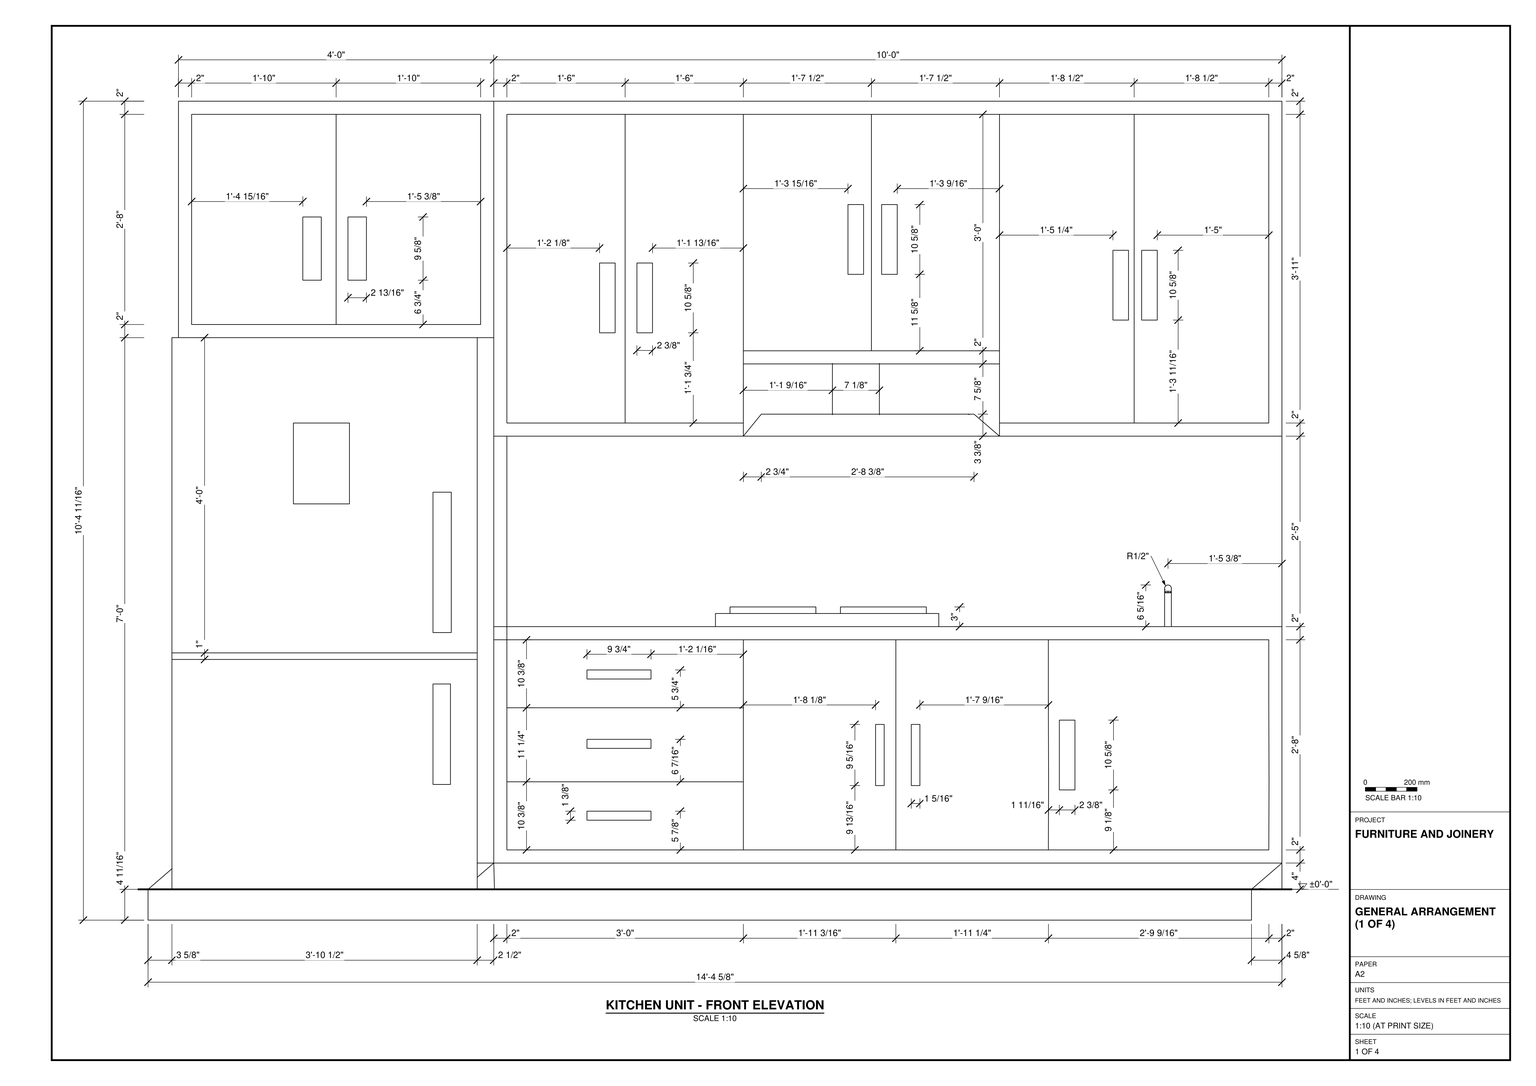
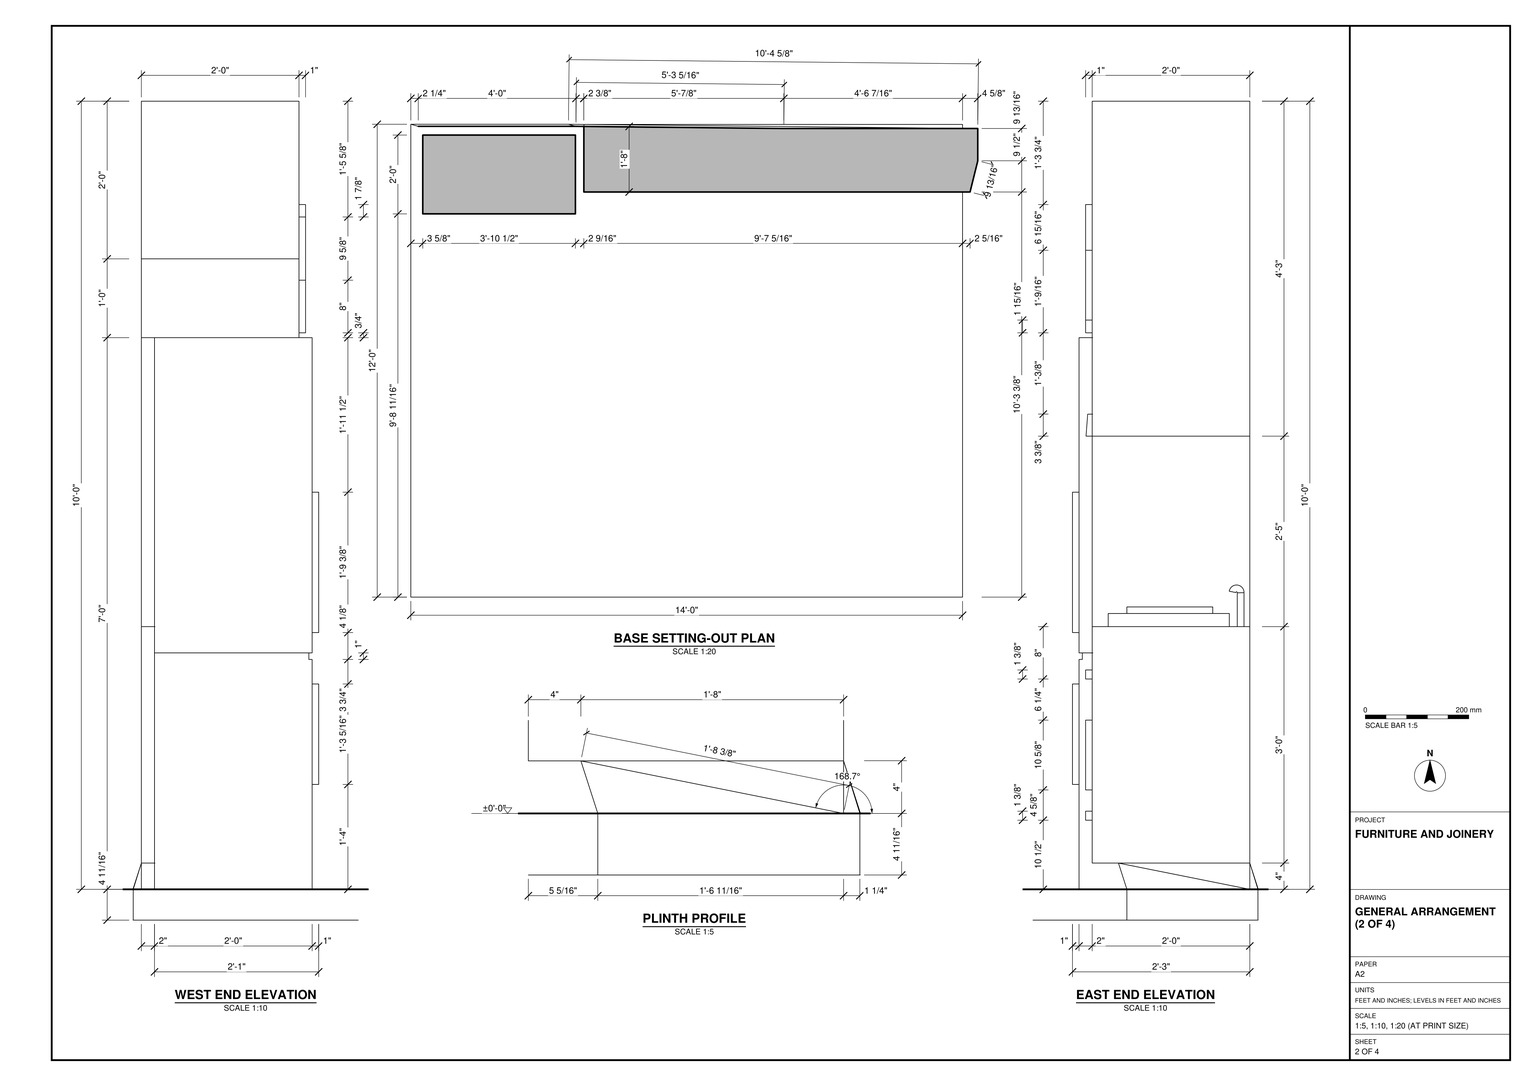
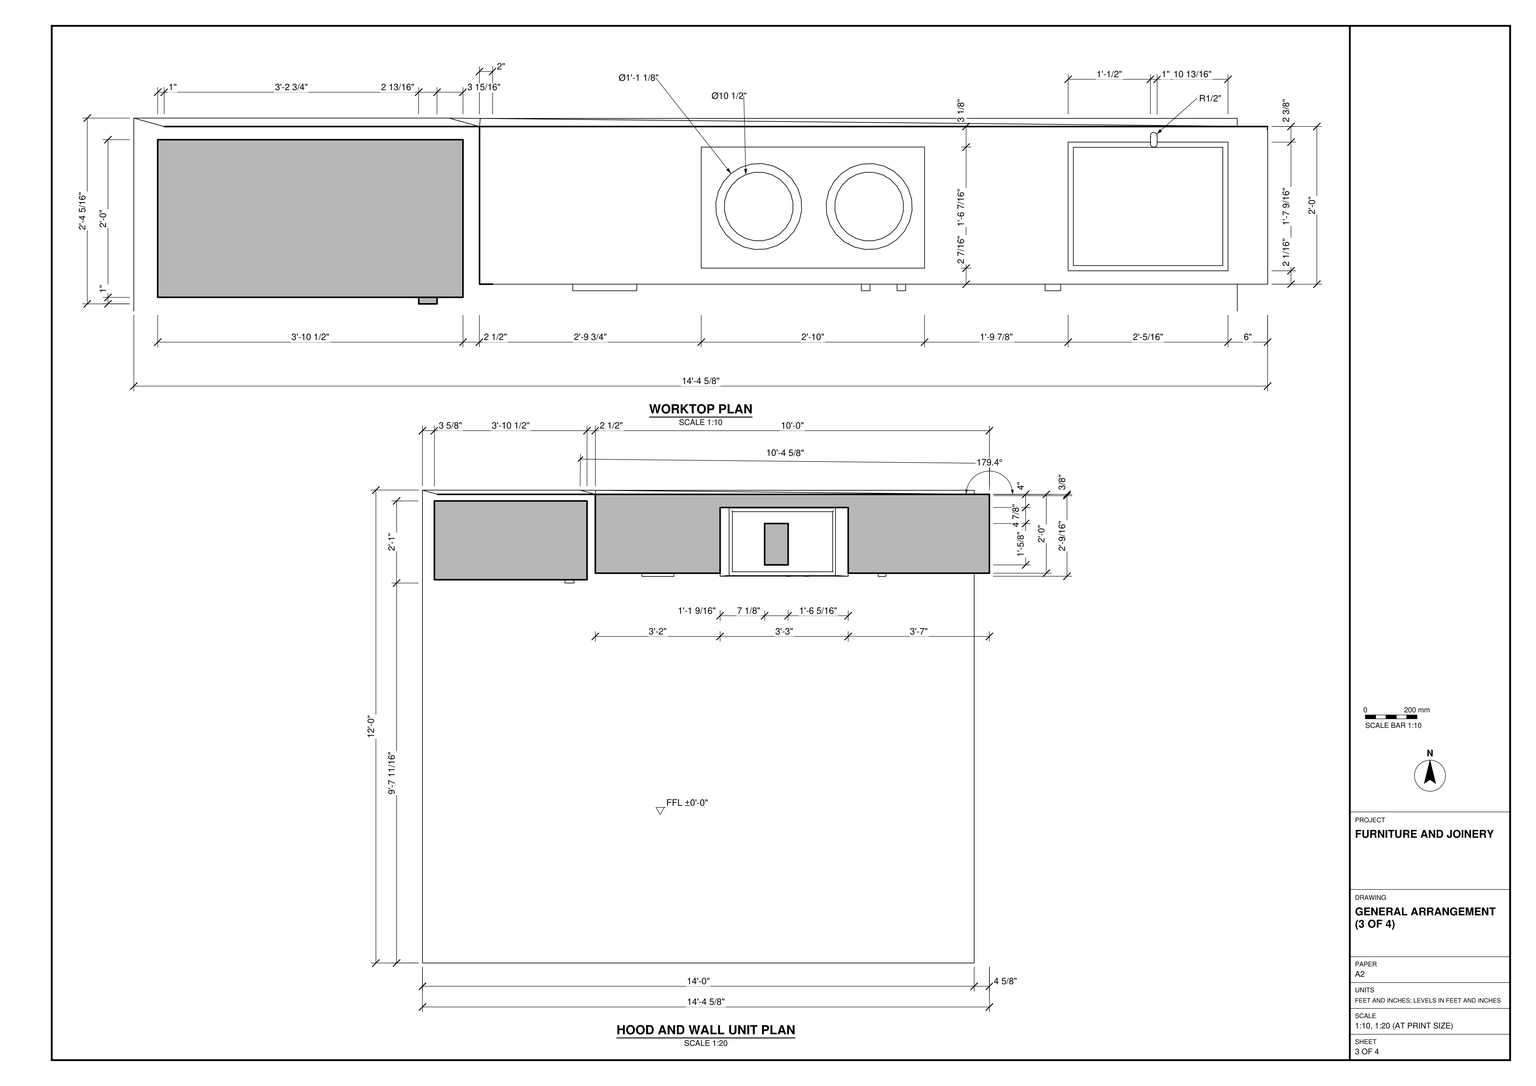
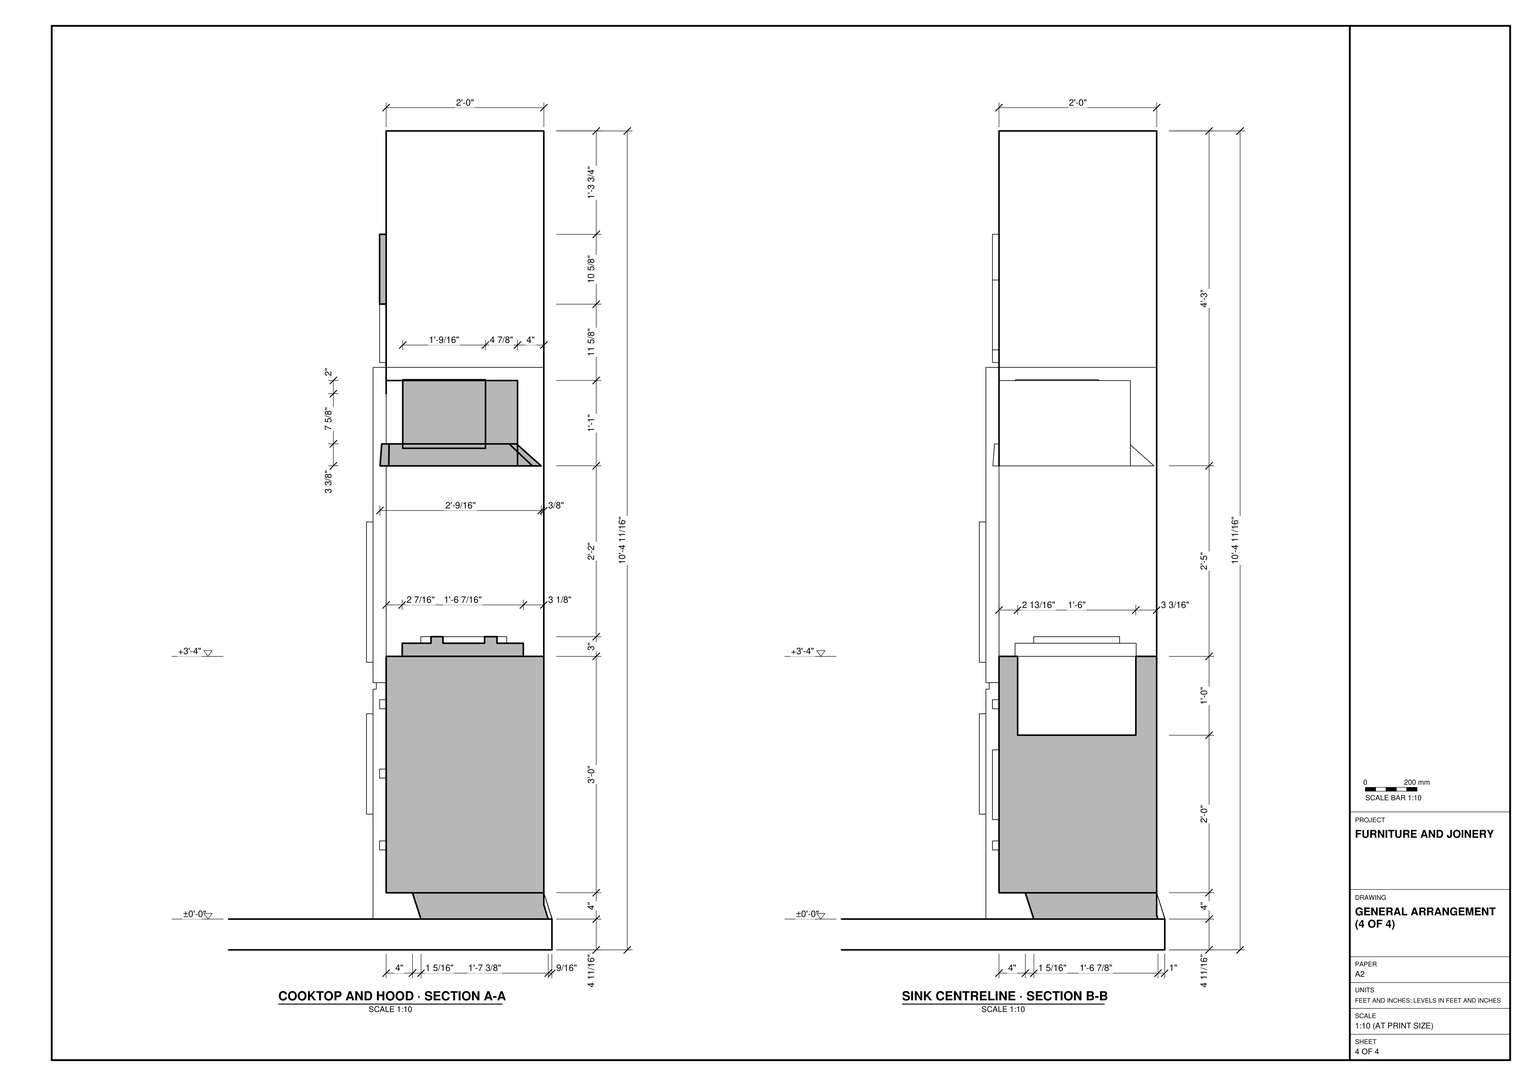
Build the kitchen unit in SketchUp from task_files/diagram_01.pdf. Work in feet and inches. The overall model is 14'-4 5/8" wide, 12'-0" deep and 10'-4 11/16" high, including the floor base. Use the single finished floor level of ±0'-0" as the datum. Set the cabinetry along the back edge of the floor base, leaving the floor in front clear.

Facing the unit, place the refrigerator on the left with a two-door cupboard above it. To its right, build the 10'-0" cabinet run on the plinth, following the sloping plinth profile in the end view. Below the worktop, place the drawer stack next to the refrigerator and the cupboard doors to the right. Follow the front elevation for the frame thicknesses, front divisions and pull positions. Fit the cooktop beneath the hood and the sink with its tap near the right end. Align the wall cupboard tops with the cupboard over the refrigerator, but shorten the middle pair of doors to leave space for the hood.

Keep the floor base and each joinery piece as separate groups or components, and use components for repeated parts such as matching pulls. Appliances, decor and loose items shown may be any suitable library components. Save one SketchUp model as output_files/kitchen_cabinet_run_with_its_worktop_and_appliances.skp.

# SketchUp Ruby script. Lengths in inches.
U = 1.inch
M = Sketchup.active_model
def pt(a) = Geom::Point3d.new(a.map { |v| v * U })
def face(e, loops, mat)
  f = e.add_face(loops[0].map { |a| pt(a) })
  loops[1..].each { |l| e.add_face(l.map { |a| pt(a) }).erase! }
  f.material = f.back_material = mat if mat
  f
end
# faces: each face lists its corners as indices into pts; further lists are holes
def faces(e, pts, list, mat = nil) = list.each { |f| face(e, (f[0].is_a?(Array) ? f : [f]).map { |l| l.map { |i| pts[i] } }, mat) }
# xy, xz, yz: faces in a plane at the given z, y or x. An outline is a flat list of corners, or four numbers for a rectangle; further outlines are holes
def ring(l) = l.size == 4 ? [[l[0], l[1]], [l[2], l[1]], [l[2], l[3]], [l[0], l[3]]] : l.each_slice(2).to_a
def flat(e, list, mat, &to3) = list.each { |f| face(e, (f[0].is_a?(Array) ? f : [f]).map { |l| ring(l).map { |u, v| to3.(u, v) } }, mat) }
def xy(e, z, list, mat = nil) = flat(e, list, mat) { |x, y| [x, y, z] }
def xz(e, y, list, mat = nil) = flat(e, list, mat) { |x, z| [x, y, z] }
def yz(e, x, list, mat = nil) = flat(e, list, mat) { |y, z| [x, y, z] }
def lines(e, pts, list) = list.each { |a, b| e.add_line(pt(pts[a]), pt(pts[b])) }
# prism: a flat outline (further loops are holes) pulled along v
def prism(e, loops, v, mat = nil)
  f = face(e, loops, mat); d = Geom::Vector3d.new(v.map { |x| x * U })
  f.pushpull(f.normal.samedirection?(d) ? d.length : -d.length)
end
def box(e, o, s, mat = nil) = prism(e, [[o, [o[0] + s[0], o[1], o[2]], [o[0] + s[0], o[1] + s[1], o[2]], [o[0], o[1] + s[1], o[2]]]], [0, 0, s[2]], mat)
def at(x, y, z, deg = 0) = Geom::Transformation.translation(pt([x, y, z])) * Geom::Transformation.rotation(ORIGIN, Z_AXIS, deg.degrees)
def axes(o, x, y, z) = Geom::Transformation.new([*x, 0, *y, 0, *z, 0, *pt(o).to_a, 1])
def part(name) = M.definitions.add(name)
# library, detail: a bought-in or finely detailed component or shape, given as its bounding box
def library(name, o, s) = part(name).tap { |d| box(d.entities, o, s) }
def detail(e, o, s) = box(e.add_group.entities, o, s)
def put(e, d, t, mat = nil) = e.add_instance(d, t).tap { |i| i.material = mat if mat }
def group(e, t, mat = nil) = e.add_group.tap { |g| g.transformation = t; g.material = mat if mat }.entities
root = M.entities
M.materials.add("[Color B08]").color = [102, 25, 0]
M.materials.add("[Color D01]").color = [255, 242, 204]
M.materials.add("[Color H08]").color = [0, 102, 102]
M.materials.add("[Color M06]").color = [86, 86, 86]
M.materials.add("[Color M08]").color = [30, 30, 30]
M.materials.add("[Color M09]").color = [0, 0, 0]
M.materials.add("[Marble Carrara Gold Floor Tile]").color = [225, 223, 217]
M.materials.add("[Wood Cherry Original]").color = [152, 86, 42]
xy(root,-4.6875,[[0,0,0,144,48,144,52.74,143.95,168,143.95,168,0]])
xy(root,0,[[0,0,168,0,168,124,52.74,124,52.74,143.95,48,144,0,144],[52.74,124,52.74,143.95,168,142.76,168,124],[168,124,168,142.76,172.64,142.71,169.26,129.1],[168,142.76,168,143.95,52.74,143.95]])
xy(root,4,[[52.64,118.71,172.64,122.71],[52.64,122.71,172.64,142.71]])
xy(root,10.53,[[66.83,117.71,76.58,118.71]],"[Color M09]")
xy(root,11.9,[[66.83,117.71,76.58,118.71]],"[Color M09]")
xy(root,15.14,[[138.75,117.71,141.125,118.71]],"[Color M09]")
xy(root,15.8,[[110.77,117.71,112.08,118.71],[116.21,117.71,117.52,118.71]],"[Color M09]")
xy(root,21.46,[[66.83,117.71,76.58,118.71]],"[Color M09]")
xy(root,22.84,[[66.83,117.71,76.58,118.71]],"[Color M09]")
xy(root,25.11,[[110.77,117.71,112.08,118.71],[116.21,117.71,117.52,118.71]],"[Color M09]")
xy(root,25.76,[[138.75,117.71,141.125,118.71]])
xy(root,28,[[143.05,121.55,165.8,139.55]])
xy(root,32.03,[[66.83,117.71,76.58,118.71]],"[Color M09]")
xy(root,33.4,[[66.83,117.71,76.58,118.71]],"[Color M09]")
xy(root,40,[[[142.25,120.75,166.59,140.34],[143.05,121.55,165.8,139.55]],[155.29,140.8,155.16,140.82,155.03,140.87,154.93,140.95,154.85,141.06,154.79,141.18,154.78,141.32,154.79,141.45,154.85,141.57,154.93,141.68,155.03,141.76,155.16,141.8125,155.29,141.83,155.42,141.8125,155.55,141.76,155.65,141.68,155.73,141.57,155.79,141.45,155.8,141.32,155.79,141.18,155.73,141.06,155.65,140.95,155.55,140.87,155.42,140.82]])
xy(root,40,[[[52.64,118.71,172.64,142.71],[142.25,120.75,166.59,140.34],[155.29,140.8,155.16,140.82,155.03,140.87,154.93,140.95,154.85,141.06,154.79,141.18,154.78,141.32,154.79,141.45,154.85,141.57,154.93,141.68,155.03,141.76,155.16,141.8125,155.29,141.83,155.42,141.8125,155.55,141.76,155.65,141.68,155.73,141.57,155.79,141.45,155.8,141.32,155.79,141.18,155.73,141.06,155.65,140.95,155.55,140.87,155.42,140.82]]],"[Marble Carrara Gold Floor Tile]")
xy(root,71.68,[[104.2,121.24,111.35,133.84]])
xy(root,82,[[90.64,118.71,129.64,138.71]])
xy(root,82.12,[[104.2,121.24,111.35,133.84]])
xy(root,84,[[4.64,118.71,52.64,142.71]])
xy(root,84.74,[[68.74,117.71,71.12,118.71],[74.43,117.71,76.81,118.71]],"[Color M09]")
xy(root,86.67,[[146.91,117.71,149.28,118.71],[151.28,117.71,153.66,118.71]],"[Color M09]")
xy(root,92.75,[[23.5625,117.71,26.375,118.71],[30.4375,117.71,33.25,118.71]],"[Color M09]")
xy(root,93.64,[[106.57,117.71,108.94,118.71],[111.69,117.71,114.07,118.71]],"[Color M09]")
xy(root,95.36,[[68.74,117.71,71.12,118.71],[74.43,117.71,76.81,118.71]],"[Color M09]")
xy(root,97.3,[[146.91,117.71,149.28,118.71],[151.28,117.71,153.66,118.71]],"[Color M09]")
xy(root,102.375,[[23.5625,117.71,26.375,118.71],[30.4375,117.71,33.25,118.71]],"[Color M09]")
xy(root,104.26,[[106.57,117.71,108.94,118.71],[111.69,117.71,114.07,118.71]],"[Color M09]")
xy(root,120,[[4.64,118.71,52.64,142.71],[52.64,118.71,172.64,142.71]],"[Color D01]")
xz(root,0,[[0,-4.6875,168,0]])
xz(root,117.71,[[66.83,10.53,76.58,11.9],[138.75,15.14,141.125,25.76],[110.77,15.8,112.08,25.11],[116.21,15.8,117.52,25.11],[66.83,21.46,76.58,22.84],
  [66.83,32.03,76.58,33.4],[68.74,84.74,71.12,95.36],[74.43,84.74,76.81,95.36],[146.91,86.67,149.28,97.3],[151.28,86.67,153.66,97.3],
  [23.5625,92.75,26.375,102.375],[30.4375,92.75,33.25,102.375],[106.57,93.64,108.94,104.26],[111.69,93.64,114.07,104.26]],"[Color M09]")
xz(root,118.71,[[66.83,10.53,76.58,11.9],[110.77,15.8,112.08,25.11],[116.21,15.8,117.52,25.11],[66.83,21.46,76.58,22.84],[66.83,32.03,76.58,33.4],
  [68.74,84.74,71.12,95.36],[74.43,84.74,76.81,95.36],[146.91,86.67,149.28,97.3],[106.57,93.64,108.94,104.26]])
xz(root,118.71,[[52.64,4,172.64,4,172.64,40,54.64,40,54.64,38,170.64,38,170.64,27.65,170.67,16.375,170.64,6,54.64,6,54.64,38,52.64,38],[52.64,69,90.64,69,90.64,71,54.64,71,54.64,118,170.64,118,170.64,71,129.64,71,129.64,69,172.64,69,172.64,120,52.64,120],[90.64,80,129.64,82],[[4.64,84,52.64,120],[6.64,86,50.64,118]]],"[Color B08]")
xz(root,118.71,[[[54.64,71,72.64,118],[68.74,84.74,71.12,95.36]],[[72.64,71,90.64,118],[74.43,84.74,76.81,95.36]],[[129.64,71,150.14,118],[146.91,86.67,149.28,97.3]],[[150.14,71,170.64,118],[151.28,86.67,153.66,97.3]],[[90.64,82,110.14,118],[106.57,93.64,108.94,104.26]],
  [[110.14,82,129.64,118],[111.69,93.64,114.07,104.26]],[[6.64,86,28.64,118],[23.5625,92.75,26.375,102.375]],[[28.64,86,50.64,118],[30.4375,92.75,33.25,102.375]]],"[Color D01]")
xz(root,118.71,[[[54.64,6,90.64,16.375],[66.83,10.53,76.58,11.9]],[[90.64,6,113.86,38],[110.77,15.8,112.08,25.11]],[[113.86,6,137.07,6,137.11,16.375,137.07,27.65,137.07,38,113.86,38],[116.21,15.8,117.52,25.11]],[[137.07,6,170.64,6,170.67,16.375,170.64,27.65,170.64,38,137.07,38,137.07,27.65,137.11,16.375],[138.75,15.14,141.125,25.76]],[[54.64,16.375,90.64,27.65],[66.83,21.46,76.58,22.84]],
  [[54.64,27.65,90.64,38],[66.83,32.03,76.58,33.4]]],"[Color H08]")
xz(root,118.71,[[52.64,38,54.64,40],[52.64,40,54.64,69]],"[Wood Cherry Original]")
xz(root,121.24,[[104.2,71.68,111.35,82.12]],"[Color M06]")
xz(root,121.55,[[143.05,28,165.8,40]])
xz(root,133.84,[[104.2,71.68,111.35,82.12]])
xz(root,138.71,[[90.64,69,129.64,82]],"[Color D01]")
xz(root,139.55,[[143.05,28,165.8,40]])
xz(root,142.71,[[172.64,0,52.64,4,172.64,4],[4.64,4,52.64,84],[52.64,4,172.64,40],[52.64,69,172.64,120],[4.64,84,52.64,120]])
xz(root,142.71,[[52.64,40,172.64,69]],"[Marble Carrara Gold Floor Tile]")
xz(root,143.95,[[52.74,-4.6875,168,0]])
xz(root,144,[[0,-4.6875,48,0]])
yz(root,0,[[0,-4.6875,144,0]])
yz(root,4.64,[[118.71,84,142.71,96],[118.71,96,142.71,120]],"[Color D01]")
yz(root,23.5625,[[117.71,92.75,118.71,102.375]],"[Color M09]")
yz(root,26.375,[[117.71,92.75,118.71,102.375]],"[Color M09]")
yz(root,30.4375,[[117.71,92.75,118.71,102.375]],"[Color M09]")
yz(root,33.25,[[117.71,92.75,118.71,102.375]],"[Color M09]")
yz(root,52.64,[[118.71,84,142.71,120]])
yz(root,52.64,[[118.71,4,142.71,40],[118.71,40,142.71,84]],"[Wood Cherry Original]")
yz(root,66.83,[[117.71,10.53,118.71,11.9],[117.71,21.46,118.71,22.84],[117.71,32.03,118.71,33.4]],"[Color M09]")
yz(root,68.74,[[117.71,84.74,118.71,95.36]],"[Color M09]")
yz(root,71.12,[[117.71,84.74,118.71,95.36]],"[Color M09]")
yz(root,74.43,[[117.71,84.74,118.71,95.36]])
yz(root,76.58,[[117.71,10.53,118.71,11.9],[117.71,21.46,118.71,22.84],[117.71,32.03,118.71,33.4]],"[Color M09]")
yz(root,76.81,[[117.71,84.74,118.71,95.36]],"[Color M09]")
yz(root,90.64,[[118.71,69,138.71,82]],"[Color D01]")
yz(root,104.2,[[121.24,71.68,133.84,82.12]])
yz(root,106.57,[[117.71,93.64,118.71,104.26]],"[Color M09]")
yz(root,108.94,[[117.71,93.64,118.71,104.26]],"[Color M09]")
yz(root,110.77,[[117.71,15.8,118.71,25.11]],"[Color M09]")
yz(root,111.35,[[121.24,71.68,133.84,82.12]])
yz(root,111.69,[[117.71,93.64,118.71,104.26]],"[Color M09]")
yz(root,112.08,[[117.71,15.8,118.71,25.11]],"[Color M09]")
yz(root,114.07,[[117.71,93.64,118.71,104.26]],"[Color M09]")
yz(root,116.21,[[117.71,15.8,118.71,25.11]],"[Color M09]")
yz(root,117.52,[[117.71,15.8,118.71,25.11]],"[Color M09]")
yz(root,129.64,[[118.71,69,138.71,82]],"[Color D01]")
yz(root,138.75,[[117.71,15.14,118.71,25.76]],"[Color M09]")
yz(root,141.125,[[117.71,15.14,118.71,25.76]],"[Color M09]")
yz(root,143.05,[[121.55,28,139.55,40]])
yz(root,146.91,[[117.71,86.67,118.71,97.3]],"[Color M09]")
yz(root,149.28,[[117.71,86.67,118.71,97.3]],"[Color M09]")
yz(root,151.28,[[117.71,86.67,118.71,97.3]],"[Color M09]")
yz(root,153.66,[[117.71,86.67,118.71,97.3]],"[Color M09]")
yz(root,165.8,[[121.55,28,139.55,40]])
yz(root,168,[[0,-4.6875,124,0],[124,-4.6875,143.95,0]])
yz(root,172.64,[[118.71,69,142.71,120]])
yz(root,172.64,[[142.71,0,142.71,4,122.71,4],[118.71,4,142.71,40]],"[Wood Cherry Original]")
p = [[48,144,0],[52.74,143.95,0],[52.74,143.95,-4.6875],[48,144,-4.6875],[172.64,122.71,4],[52.64,122.71,4],
  [52.74,124,0],[168,124,0],[52.64,142.71,4],[169.26,129.1,0],[172.64,142.71,0],[0,144,0],
  [4.64,142.71,4],[168,142.76,0],[155.03,140.87,40],[155.16,140.82,40],[155.16,140.82,45.15],[155.03,140.87,45.15],
  [155.29,140.8,40],[155.29,140.8,45.15],[155.42,140.82,40],[155.42,140.82,45.15],[155.55,140.87,40],[155.55,140.87,45.15],
  [154.93,140.95,40],[154.93,140.95,45.15],[155.65,140.95,40],[155.65,140.95,45.15],[154.85,141.06,40],[154.85,141.06,45.16],
  [155.73,141.06,40],[155.73,141.06,45.16],[154.79,141.18,40],[154.79,141.18,45.16],[155.79,141.18,40],[155.79,141.18,45.16],
  [154.78,141.32,40],[154.78,141.32,45.16],[155.8,141.32,40],[155.8,141.32,45.16],[154.79,141.45,40],[154.79,141.45,45.17],
  [155.79,141.45,40],[155.79,141.45,45.17],[154.85,141.57,40],[154.85,141.57,45.17],[155.73,141.57,40],[155.73,141.57,45.17],
  [154.93,141.68,40],[154.93,141.68,45.17],[155.65,141.68,40],[155.65,141.68,45.17],[155.03,141.76,40],[155.03,141.76,45.18],
  [155.55,141.76,40],[155.55,141.76,45.18],[155.16,141.8125,40],[155.16,141.8125,45.18],[155.29,141.83,40],[155.29,141.83,45.18],
  [155.42,141.8125,40],[155.42,141.8125,45.18],[155.16,140.8125,45.23],[155.03,140.87,45.24],[155.29,140.8,45.23],[155.42,140.8125,45.23],
  [155.55,140.87,45.24],[154.93,140.95,45.26],[155.65,140.95,45.26],[154.93,140.4375,45.22],[155.03,140.52,45.2],[155.16,140.57,45.19],
  [155.29,140.59,45.1875],[155.42,140.57,45.19],[155.55,140.52,45.2],[155.65,140.4375,45.22],[155.73,140.33,45.24],[155.79,140.21,45.26],
  [155.8,140.08,45.29],[155.79,139.95,45.32],[155.73,139.83,45.34],[155.65,139.73,45.36],[155.55,139.65,45.38],[155.42,139.6,45.39],
  [155.29,139.58,45.39],[155.16,139.6,45.39],[155.03,139.65,45.38],[154.93,139.73,45.36],[154.85,139.83,45.34],[154.79,139.95,45.32],
  [154.78,140.08,45.29],[154.79,140.21,45.26],[154.85,140.33,45.24],[154.79,140.23,45.37],[154.85,140.35,45.32],[155.73,140.35,45.32],
  [155.79,140.23,45.37],[154.93,140.45,45.29],[155.65,140.45,45.29],[155.03,140.53,45.26],[155.55,140.53,45.26],[155.03,140.55,45.3],
  [155.16,140.59,45.27],[155.16,140.58,45.25],[155.42,140.59,45.27],[155.55,140.55,45.3],[155.42,140.58,45.25],[155.29,140.61,45.26],
  [155.29,140.6,45.24],[155.16,140.8,45.26],[155.03,140.85,45.28],[155.29,140.79,45.25],[155.42,140.8,45.26],[155.55,140.85,45.28],
  [154.85,141.05,45.28],[154.93,140.92,45.32],[155.65,140.92,45.32],[155.73,141.05,45.28],[154.79,141.17,45.3],[155.79,141.17,45.3],
  [154.78,141.31,45.33],[155.8,141.31,45.33],[154.79,141.4375,45.35],[155.79,141.4375,45.35],[154.85,141.56,45.375],[155.73,141.56,45.375],
  [154.93,141.66,45.4],[155.65,141.66,45.4],[155.03,141.75,45.41],[155.16,141.8,45.42],[155.42,141.8,45.42],[155.55,141.75,45.41],
  [155.29,141.8125,45.42],[154.93,139.76,45.53],[154.85,139.86,45.49],[155.73,139.86,45.49],[155.65,139.76,45.53],[154.79,139.98,45.45],
  [155.79,139.98,45.45],[154.78,140.11,45.41],[155.8,140.11,45.41],[154.79,140.29,45.48],[154.85,140.39,45.41],[155.73,140.39,45.41],
  [155.79,140.29,45.48],[154.85,140.46,45.48],[154.93,140.53,45.4],[154.93,140.48,45.35],[155.65,140.53,45.4],[155.73,140.46,45.48],
  [155.65,140.48,45.35],[154.93,140.58,45.4375],[155.03,140.62,45.36],[155.03,140.58,45.34],[155.55,140.62,45.36],[155.65,140.58,45.4375],
  [155.55,140.58,45.34],[155.03,140.66,45.375],[155.16,140.67,45.33],[155.16,140.64,45.32],[155.16,140.62,45.3],[155.29,140.67,45.31],
  [155.29,140.65,45.3],[155.29,140.625,45.29],[155.42,140.67,45.33],[155.42,140.64,45.32],[155.42,140.62,45.3],[155.55,140.66,45.375],
  [155.03,140.79,45.35],[155.16,140.76,45.31],[155.16,140.73,45.32],[155.03,140.75,45.37],[155.16,140.7,45.33],[155.03,140.71,45.38],
  [155.29,140.75,45.29],[155.29,140.73,45.31],[155.29,140.7,45.3125],[155.42,140.76,45.31],[155.42,140.73,45.32],[155.42,140.7,45.33],
  [155.55,140.79,45.35],[155.55,140.75,45.37],[155.55,140.71,45.38],[155.03,140.83,45.32],[154.93,140.89,45.375],[154.93,140.84,45.42],
  [155.16,140.79,45.29],[155.29,140.77,45.28],[155.42,140.79,45.29],[155.55,140.83,45.32],[155.65,140.89,45.375],[155.65,140.84,45.42],
  [154.85,141.02,45.37],[154.85,140.97,45.44],[155.73,141.02,45.37],[155.73,140.97,45.44],[154.79,141.13,45.42],[155.79,141.13,45.42],
  [154.78,141.25,45.48],[155.8,141.25,45.48],[154.79,141.375,45.54],[155.79,141.375,45.54],[155.03,139.68,45.55],[155.16,139.63,45.57],
  [155.29,139.62,45.58],[155.42,139.63,45.57],[155.55,139.68,45.55],[154.79,140.07,45.63],[154.78,140.18,45.55],[155.8,140.18,45.55],
  [155.79,140.07,45.63],[154.79,140.375,45.57],[155.79,140.375,45.57],[154.85,140.625,45.5625],[154.93,140.65,45.46],[154.85,140.54,45.53],
  [155.65,140.65,45.46],[155.73,140.625,45.5625],[155.73,140.54,45.53],[154.93,140.71,45.46],[155.65,140.71,45.46],[154.85,140.8125,45.55],
  [154.93,140.78,45.45],[154.85,140.72,45.57],[155.65,140.78,45.45],[155.73,140.8125,45.55],[155.73,140.72,45.57],[154.85,140.9,45.51],
  [155.73,140.9,45.51],[154.79,141.0625,45.53],[154.79,140.97,45.61],[155.79,141.0625,45.53],[155.79,140.97,45.61],[154.78,141.16,45.61],
  [155.8,141.16,45.61],[154.85,141.49,45.59],[155.73,141.49,45.59],[154.93,141.58,45.64],[155.65,141.58,45.64],[155.03,141.66,45.68],
  [155.55,141.66,45.68],[155.16,141.7,45.7],[155.29,141.72,45.71],[155.42,141.7,45.7],[155.03,139.81,45.81],[154.93,139.875,45.76],
  [155.65,139.875,45.76],[155.55,139.81,45.81],[154.85,139.96,45.7],[155.73,139.96,45.7],[154.78,140.29,45.68],[155.8,140.29,45.68],
  [154.79,140.48,45.65],[155.79,140.48,45.65],[154.79,140.6,45.6875],[155.79,140.6,45.6875],[154.79,140.85,45.67],[154.79,140.73,45.69],
  [155.79,140.85,45.67],[155.79,140.73,45.69],[154.78,141.04,45.72],[155.8,141.04,45.72],[154.79,141.27,45.7],[155.79,141.27,45.7],
  [154.85,141.36,45.78],[155.73,141.36,45.78],[155.16,139.76,45.83],[155.29,139.75,45.84],[155.42,139.76,45.83],[154.85,140.12,45.87],
  [154.79,140.2,45.78],[155.79,140.2,45.78],[155.73,140.12,45.87],[154.78,140.42,45.77],[155.8,140.42,45.77],[154.78,140.58,45.82],
  [155.8,140.58,45.82],[154.78,140.9,45.79],[155.8,140.9,45.79],[154.79,141.12,45.83],[155.79,141.12,45.83],[154.93,141.44,45.86],
  [155.03,141.5,45.91],[155.55,141.5,45.91],[155.65,141.44,45.86],[154.93,140.05,45.95],[155.65,140.05,45.95],[154.79,140.36,45.89],
  [155.79,140.36,45.89],[154.78,140.74,45.83],[155.8,140.74,45.83],[154.79,140.94,45.92],[155.79,140.94,45.92],[154.85,141.1875,45.9375],
  [155.73,141.1875,45.9375],[155.16,141.54,45.94],[155.29,141.55,45.95],[155.42,141.54,45.94],[155.29,139.95,46.07],[155.16,139.96,46.05],
  [155.42,139.96,46.05],[155.03,139.99,46.01],[155.55,139.99,46.01],[154.85,140.31,46],[155.73,140.31,46],[154.79,140.55,45.95],
  [155.79,140.55,45.95],[154.79,140.75,45.96],[155.79,140.75,45.96],[154.85,140.98,46.04],[155.73,140.98,46.04],[154.93,141.25,46.03],
  [155.65,141.25,46.03],[154.93,140.26,46.09],[155.65,140.26,46.09],[154.85,140.53,46.07],[155.73,140.53,46.07],[154.85,140.76,46.09],
  [155.73,140.76,46.09],[154.93,141.02,46.14],[155.65,141.02,46.14],[155.03,141.29,46.09],[155.55,141.29,46.09],[155.16,141.32,46.14],
  [155.29,141.33,46.15],[155.42,141.32,46.14],[155.03,140.23,46.17],[155.16,140.2,46.22],[155.55,140.23,46.17],[155.42,140.2,46.22],
  [154.93,140.51,46.18],[155.65,140.51,46.18],[154.93,140.76,46.19],[155.65,140.76,46.19],[155.03,141.04,46.22],[155.55,141.04,46.22],
  [155.29,140.19,46.23],[155.03,140.49,46.26],[155.55,140.49,46.26],[155.03,140.77,46.27],[155.55,140.77,46.27],[155.16,141.06,46.27],
  [155.42,141.06,46.27],[155.29,141.07,46.28],[155.16,140.48,46.31],[155.29,140.48,46.33],[155.42,140.48,46.31],[155.16,140.77,46.33],
  [155.42,140.77,46.33],[155.29,140.77,46.34],[4.64,142.71,0],[155.29,141.32,40],[155.29,141.32,45.16],[155.29,141.31,45.33],
  [155.29,141.25,45.48],[155.29,141.16,45.61],[155.29,141.04,45.72],[155.29,140.9,45.79],[155.29,140.74,45.83],[155.29,140.58,45.82],
  [155.29,140.42,45.77],[155.29,140.29,45.68],[155.29,140.18,45.55],[155.29,140.11,45.41],[155.29,140.07,45.25],[155.29,141.32,45.25]]
faces(root,p,[[0,1,2,3],[8,1,6,5],[9,10,4,7],[11,12,8,0],[0,8,1],[13,1,8,10],[14,15,16,17],[15,18,19,16],
  [18,20,21,19],[20,22,23,21],[24,14,17,25],[22,26,27,23],[28,24,25,29],[26,30,31,27],[32,28,29,33],[30,34,35,31],
  [36,32,33,37],[34,38,39,35],[40,36,37,41],[38,42,43,39],[44,40,41,45],[42,46,47,43],[48,44,45,49],[46,50,51,47],
  [52,48,49,53],[50,54,55,51],[56,52,53,57],[58,56,57,59],[60,58,59,61],[54,60,61,55],[17,16,62,63],[16,19,64,62],
  [19,21,65,64],[21,23,66,65],[25,17,63,67],[23,27,68,66],[69,70,71,72,73,74,75,76,77,78,79,80,81,82,83,84,85,86,87,88,89,90,91,92],[93,94,92,91],[95,96,77,76],[94,97,69,92],
  [98,95,76,75],[97,99,70,69],[100,98,75,74],[101,102,103,99],[99,103,71,70],[104,105,100,106],[106,100,74,73],[102,107,108,103],
  [103,108,72,71],[107,104,106,108],[108,106,73,72],[63,62,109,110],[62,64,111,109],[64,65,112,111],[65,66,113,112],[29,25,67,114],
  [67,63,110,115],[66,68,116,113],[27,31,117,68],[33,29,114,118],[31,35,119,117],[37,33,118,120],[35,39,121,119],[41,37,120,122],
  [39,43,123,121],[45,41,122,124],[43,47,125,123],[49,45,124,126],[47,51,127,125],[53,49,126,128],[57,53,128,129],[55,61,130,131],
  [51,55,131,127],[59,57,129,132],[61,59,132,130],[133,134,88,87],[135,136,81,80],[134,137,89,88],[138,135,80,79],[137,139,90,89],
  [140,138,79,78],[139,93,91,90],[96,140,78,77],[141,142,94,93],[143,144,96,95],[145,146,147,142],[142,147,97,94],[148,149,143,150],
  [150,143,95,98],[151,152,153,146],[146,153,101,147],[147,101,99,97],[154,155,148,156],[156,148,150,105],[105,150,98,100],[157,158,159,152],
  [152,159,160,153],[153,160,102,101],[158,161,162,159],[159,162,163,160],[160,163,107,102],[161,164,165,162],[162,165,166,163],[163,166,104,107],
  [164,167,154,165],[165,154,156,166],[166,156,105,104],[168,169,170,171],[171,170,172,173],[173,172,158,157],[169,174,175,170],[170,175,176,172],
  [172,176,161,158],[174,177,178,175],[175,178,179,176],[176,179,164,161],[177,180,181,178],[178,181,182,179],[179,182,167,164],[115,110,183,184],
  [184,183,168,185],[110,109,186,183],[183,186,169,168],[109,111,187,186],[186,187,174,169],[111,112,188,187],[187,188,177,174],[112,113,189,188],
  [188,189,180,177],[113,116,190,189],[189,190,191,180],[114,67,115,192],[192,115,184,193],[68,117,194,116],[116,194,195,190],[118,114,192,196],
  [117,119,197,194],[120,118,196,198],[119,121,199,197],[122,120,198,200],[121,123,201,199],[202,133,87,86],[203,202,86,85],[204,203,85,84],
  [205,204,84,83],[206,205,83,82],[136,206,82,81],[207,208,139,137],[209,210,138,140],[208,141,93,139],[144,209,140,96],[211,145,142,141],
  [149,212,144,143],[213,214,151,215],[215,151,146,145],[216,217,218,155],[155,218,149,148],[219,173,157,214],[214,157,152,151],[182,220,216,167],
  [167,216,155,154],[221,222,219,223],[222,171,173,219],[181,224,220,182],[224,225,226,220],[193,184,185,227],[227,185,222,221],[185,168,171,222],
  [180,191,224,181],[190,195,228,191],[191,228,225,224],[229,193,227,230],[195,231,232,228],[196,192,193,229],[194,197,231,195],[198,196,229,233],
  [197,199,234,231],[124,122,200,235],[123,125,236,201],[126,124,235,237],[125,127,238,236],[128,126,237,239],[127,131,240,238],[129,128,239,241],
  [132,129,241,242],[130,132,242,243],[131,130,243,240],[244,245,133,202],[246,247,206,136],[245,248,134,133],[249,246,136,135],[248,207,137,134],
  [210,249,135,138],[250,211,141,208],[212,251,209,144],[252,215,145,211],[218,253,212,149],[254,213,215,252],[217,255,253,218],[223,219,214,213],
  [220,226,217,216],[256,221,223,257],[225,258,259,226],[230,227,221,256],[228,232,258,225],[233,229,230,260],[231,234,261,232],[200,198,233,262],
  [199,201,263,234],[235,200,262,264],[201,236,265,263],[266,244,202,203],[267,266,203,204],[268,267,204,205],[247,268,205,206],[269,270,207,248],
  [271,272,249,210],[270,250,208,207],[251,271,210,209],[273,252,211,250],[253,274,251,212],[275,254,252,273],[255,276,274,253],[257,223,213,254],
  [226,259,255,217],[260,230,256,277],[232,261,278,258],[262,233,260,279],[234,263,280,261],[237,235,264,281],[239,237,281,282],[238,240,283,284],
  [236,238,284,265],[285,269,248,245],[272,286,246,249],[287,273,250,270],[274,288,271,251],[289,257,254,275],[259,290,276,255],[277,256,257,289],
  [258,278,290,259],[279,260,277,291],[261,280,292,278],[264,262,279,293],[263,265,294,280],[241,239,282,295],[242,241,295,296],[243,242,296,297],
  [240,243,297,283],[298,299,266,267],[300,298,267,268],[301,285,245,244],[299,301,244,266],[302,300,268,247],[286,302,247,246],[303,287,270,269],
  [288,304,272,271],[305,275,273,287],[276,306,288,274],[307,289,275,305],[290,308,306,276],[291,277,289,307],[278,292,308,290],[293,279,291,309],
  [280,294,310,292],[281,264,293,311],[265,284,312,294],[313,303,269,285],[304,314,286,272],[315,305,287,303],[306,316,304,288],[317,307,305,315],
  [308,318,316,306],[309,291,307,317],[292,310,318,308],[311,293,309,319],[294,312,320,310],[282,281,311,321],[284,283,322,312],[295,282,321,323],
  [296,295,323,324],[297,296,324,325],[283,297,325,322],[326,313,285,301],[327,326,301,299],[328,329,300,302],[314,328,302,286],[330,315,303,313],
  [316,331,314,304],[319,309,317,332],[310,320,333,318],[321,311,319,334],[312,322,335,320],[336,327,299,298],[329,336,298,300],[337,330,313,326],
  [331,338,328,314],[332,317,315,330],[318,333,331,316],[334,319,332,339],[320,335,340,333],[323,321,334,341],[322,325,342,335],[324,323,341,343],
  [325,324,343,342],[344,337,326,327],[345,344,327,336],[346,345,336,329],[338,346,329,328],[339,332,330,337],[333,340,338,331],[341,334,339,347],
  [335,342,348,340],[347,339,337,344],[349,347,344,345],[348,349,345,346],[340,348,346,338],[343,341,347,349],[342,343,349,348]])
faces(root,p,[[4,5,6,7]],"[Wood Cherry Original]")
lines(root,p,[[12,350],[351,352],[352,353],[353,354],[354,355],[355,356],[356,357],[357,358],[358,359],[359,360],[360,361],[361,362],
  [362,363],[363,364],[352,365]])
g1 = group(root,at(90.64,117.77,69),"[Color M08]")
xy(g1,0,[[[0,0,39,24.54],[1.32,1.34,37.68,23.2]],[1.32,1.34,37.68,23.2]])
xy(g1,3.35,[[[2.73,0.25,35.12,20.78],[3.76,1.375,34.27,19.66]],[3.76,1.375,34.27,19.66]])
p = [[39,0,0],[35.12,0.25,3.35],[2.73,0.25,3.35],[0,0,0],[2.73,20.78,3.35],[0,24.54,0],
  [39,24.54,0],[35.12,20.78,3.35],[1.32,1.34,0],[3.76,1.375,3.35],[34.27,1.375,3.35],[37.68,1.34,0],
  [1.32,23.2,0],[3.76,19.66,3.35],[3.76,2.46,3.35],[34.27,19.66,3.35],[37.68,23.2,0]]
faces(g1,p,[[0,1,2,3],[3,2,4,5],[1,0,6,7],[8,9,10,11],[8,12,13,14,9],[15,16,11,10],[12,16,15,13],[5,4,7,6]])
g2 = group(root,at(3.64,115.71,0),"[Color M06]")
xy(g2,0,[[0,1,46.48,25]])
xy(g2,15.97,[[39.75,0,42.41,1]])
xy(g2,31.27,[[39.75,0,42.41,1]])
xy(g2,35,[[0,1,46.48,1.5]])
xy(g2,36,[[0,1,46.48,1.5],[0,1.5,46.48,25]])
xy(g2,39.1,[[39.75,0,42.53,1]])
xy(g2,60.47,[[39.75,0,42.53,1]])
xy(g2,84,[[0,1,46.48,25]])
xz(g2,0,[[39.75,15.97,42.41,31.27],[39.75,39.1,42.53,60.47]])
xz(g2,1,[[[0,0,46.48,35],[39.75,15.97,42.41,31.27]],[39.75,15.97,42.41,31.27],[[0,36,46.48,84],[18.49,58.6875,27.03,71],[39.75,39.1,42.53,60.47]],[39.75,39.1,42.53,60.47],[18.49,58.6875,27.03,71]])
xz(g2,1.5,[[0,35,46.48,36]])
xz(g2,25,[[0,0,46.48,36],[0,36,46.48,84]])
yz(g2,0,[[1,0,1,35,1.5,35,1.5,36,25,36,25,0],[1,36,25,84]])
yz(g2,39.75,[[0,15.97,1,31.27],[0,39.1,1,60.47]])
yz(g2,42.41,[[0,15.97,1,31.27]])
yz(g2,42.53,[[0,39.1,1,60.47]])
yz(g2,46.48,[[1,0,25,0,25,36,1.5,36,1.5,35,1,35],[1,36,25,84]])
g3 = group(root,at(86.39,121.15,40))
xy(g3,0,[[0,0,34,18.4375]])
xy(g3,2,[[[0,0,34,18.4375],[8.17,2.84,6.5,3.21,4.98,4.01,3.72,5.16,2.8,6.61,2.29,8.25,2.22,9.96,2.59,11.63,3.38,13.15,4.54,14.41,5.99,15.33,7.62,15.84,9.33,15.91,11,15.54,12.52,14.75,13.78,13.59,14.7,12.14,15.22,10.51,15.29,8.8,14.92,7.125,14.125,5.61,12.96,4.35,11.52,3.43,9.88,2.91],[24.99,2.84,23.3125,3.21,21.79,4.01,20.53,5.16,19.61,6.61,19.1,8.25,19.03,9.96,19.4,11.63,20.19,13.15,21.35,14.41,22.8,15.33,24.43,15.84,26.14,15.91,27.82,15.54,29.33,14.75,30.6,13.59,31.52,12.14,32.03,10.51,32.1,8.8,31.73,7.125,30.9375,5.61,29.78,4.35,28.33,3.43,26.7,2.91]],[9.39,4.17,10.72,4.51,11.91,5.18,12.89,6.15,13.58,7.33,13.95,8.65,13.96,10.02,13.62,11.34,12.94,12.54,11.98,13.51,10.8,14.21,9.48,14.58,8.11,14.59,6.78,14.25,5.59,13.57,4.61,12.61,3.92,11.43,3.55,10.11,3.54,8.74,3.88,7.41,4.56,6.22,5.52,5.24,6.7,4.54,8.02,4.18],[26.2,4.17,27.53,4.51,28.72,5.18,29.7,6.15,30.4,7.33,30.76,8.65,30.78,10.02,30.43,11.34,29.76,12.54,28.8,13.51,27.62,14.21,26.29,14.58,24.92,14.59,23.6,14.25,22.4,13.57,21.43,12.61,20.73,11.43,20.37,10.11,20.35,8.74,20.7,7.41,21.37,6.22,22.33,5.24,23.51,4.54,24.83,4.18]])
xy(g3,3,[[[8.17,2.84,9.88,2.91,11.52,3.43,12.96,4.35,14.125,5.61,14.92,7.125,15.29,8.8,15.22,10.51,14.7,12.14,13.78,13.59,12.52,14.75,11,15.54,9.33,15.91,7.62,15.84,5.99,15.33,4.54,14.41,3.38,13.15,2.59,11.63,2.22,9.96,2.29,8.25,2.8,6.61,3.72,5.16,4.98,4.01,6.5,3.21],[9.39,4.17,8.02,4.18,6.7,4.54,5.52,5.24,4.56,6.22,3.88,7.41,3.54,8.74,3.55,10.11,3.92,11.43,4.61,12.61,5.59,13.57,6.78,14.25,8.11,14.59,9.48,14.58,10.8,14.21,11.98,13.51,12.94,12.54,13.62,11.34,13.96,10.02,13.95,8.65,13.58,7.33,12.89,6.15,11.91,5.18,10.72,4.51]],[[24.99,2.84,26.7,2.91,28.33,3.43,29.78,4.35,30.9375,5.61,31.73,7.125,32.1,8.8,32.03,10.51,31.52,12.14,30.6,13.59,29.33,14.75,27.82,15.54,26.14,15.91,24.43,15.84,22.8,15.33,21.35,14.41,20.19,13.15,19.4,11.63,19.03,9.96,19.1,8.25,19.61,6.61,20.53,5.16,21.79,4.01,23.3125,3.21],[26.2,4.17,24.83,4.18,23.51,4.54,22.33,5.24,21.37,6.22,20.7,7.41,20.35,8.74,20.37,10.11,20.73,11.43,21.43,12.61,22.4,13.57,23.6,14.25,24.92,14.59,26.29,14.58,27.62,14.21,28.8,13.51,29.76,12.54,30.43,11.34,30.78,10.02,30.76,8.65,30.4,7.33,29.7,6.15,28.72,5.18,27.53,4.51]]])
xz(g3,0,[[0,0,34,2]])
xz(g3,18.4375,[[0,0,34,2]])
yz(g3,0,[[0,0,18.4375,2]])
yz(g3,34,[[0,0,18.4375,2]])
p = [[6.5,3.21,2],[8.17,2.84,2],[8.17,2.84,3],[6.5,3.21,3],[9.88,2.91,2],[9.88,2.91,3],
  [23.3125,3.21,2],[24.99,2.84,2],[24.99,2.84,3],[23.3125,3.21,3],[26.7,2.91,2],[26.7,2.91,3],
  [11.52,3.43,2],[11.52,3.43,3],[28.33,3.43,2],[28.33,3.43,3],[4.98,4.01,2],[4.98,4.01,3],
  [21.79,4.01,2],[21.79,4.01,3],[12.96,4.35,2],[12.96,4.35,3],[29.78,4.35,2],[29.78,4.35,3],
  [3.72,5.16,2],[3.72,5.16,3],[20.53,5.16,2],[20.53,5.16,3],[8.02,4.18,2],[6.7,4.54,2],
  [6.7,4.54,3],[8.02,4.18,3],[9.39,4.17,2],[9.39,4.17,3],[10.72,4.51,2],[10.72,4.51,3],
  [24.83,4.18,2],[23.51,4.54,2],[23.51,4.54,3],[24.83,4.18,3],[26.2,4.17,2],[26.2,4.17,3],
  [27.53,4.51,2],[27.53,4.51,3],[14.125,5.61,2],[14.125,5.61,3],[30.9375,5.61,2],[30.9375,5.61,3],
  [5.52,5.24,2],[5.52,5.24,3],[11.91,5.18,2],[11.91,5.18,3],[22.33,5.24,2],[22.33,5.24,3],
  [28.72,5.18,2],[28.72,5.18,3],[2.8,6.61,2],[2.8,6.61,3],[4.56,6.22,2],[4.56,6.22,3],
  [12.89,6.15,2],[12.89,6.15,3],[19.61,6.61,2],[19.61,6.61,3],[21.37,6.22,2],[21.37,6.22,3],
  [29.7,6.15,2],[29.7,6.15,3],[14.92,7.125,2],[14.92,7.125,3],[31.73,7.125,2],[31.73,7.125,3],
  [13.58,7.33,2],[13.58,7.33,3],[30.4,7.33,2],[30.4,7.33,3],[3.88,7.41,2],[3.88,7.41,3],
  [20.7,7.41,2],[20.7,7.41,3],[2.29,8.25,2],[2.29,8.25,3],[19.1,8.25,2],[19.1,8.25,3],
  [15.29,8.8,2],[15.29,8.8,3],[32.1,8.8,2],[32.1,8.8,3],[13.95,8.65,2],[13.95,8.65,3],
  [30.76,8.65,2],[30.76,8.65,3],[3.54,8.74,2],[3.54,8.74,3],[20.35,8.74,2],[20.35,8.74,3],
  [2.22,9.96,2],[2.22,9.96,3],[19.03,9.96,2],[19.03,9.96,3],[13.96,10.02,2],[13.96,10.02,3],
  [30.78,10.02,2],[30.78,10.02,3],[3.55,10.11,2],[3.55,10.11,3],[20.37,10.11,2],[20.37,10.11,3],
  [15.22,10.51,2],[15.22,10.51,3],[32.03,10.51,2],[32.03,10.51,3],[2.59,11.63,2],[2.59,11.63,3],
  [13.62,11.34,2],[13.62,11.34,3],[19.4,11.63,2],[19.4,11.63,3],[30.43,11.34,2],[30.43,11.34,3],
  [3.92,11.43,2],[3.92,11.43,3],[20.73,11.43,2],[20.73,11.43,3],[14.7,12.14,2],[14.7,12.14,3],
  [31.52,12.14,2],[31.52,12.14,3],[12.94,12.54,2],[12.94,12.54,3],[29.76,12.54,2],[29.76,12.54,3],
  [4.61,12.61,2],[4.61,12.61,3],[21.43,12.61,2],[21.43,12.61,3],[3.38,13.15,2],[3.38,13.15,3],
  [20.19,13.15,2],[20.19,13.15,3],[13.78,13.59,2],[13.78,13.59,3],[30.6,13.59,2],[30.6,13.59,3],
  [11.98,13.51,2],[11.98,13.51,3],[28.8,13.51,2],[28.8,13.51,3],[5.59,13.57,2],[5.59,13.57,3],
  [22.4,13.57,2],[22.4,13.57,3],[4.54,14.41,2],[4.54,14.41,3],[21.35,14.41,2],[21.35,14.41,3],
  [10.8,14.21,2],[10.8,14.21,3],[27.62,14.21,2],[27.62,14.21,3],[6.78,14.25,2],[6.78,14.25,3],
  [12.52,14.75,2],[12.52,14.75,3],[23.6,14.25,2],[23.6,14.25,3],[29.33,14.75,2],[29.33,14.75,3],
  [8.11,14.59,2],[8.11,14.59,3],[9.48,14.58,2],[9.48,14.58,3],[24.92,14.59,2],[24.92,14.59,3],
  [26.29,14.58,2],[26.29,14.58,3],[5.99,15.33,2],[5.99,15.33,3],[22.8,15.33,2],[22.8,15.33,3],
  [11,15.54,2],[11,15.54,3],[27.82,15.54,2],[27.82,15.54,3],[7.62,15.84,2],[7.62,15.84,3],
  [24.43,15.84,2],[24.43,15.84,3],[9.33,15.91,2],[9.33,15.91,3],[26.14,15.91,2],[26.14,15.91,3]]
faces(g3,p,[[0,1,2,3],[1,4,5,2],[6,7,8,9],[7,10,11,8],[4,12,13,5],[10,14,15,11],[16,0,3,17],[18,6,9,19],
  [12,20,21,13],[14,22,23,15],[24,16,17,25],[26,18,19,27],[28,29,30,31],[32,28,31,33],[34,32,33,35],[36,37,38,39],
  [40,36,39,41],[42,40,41,43],[20,44,45,21],[22,46,47,23],[29,48,49,30],[50,34,35,51],[37,52,53,38],[54,42,43,55],
  [56,24,25,57],[48,58,59,49],[60,50,51,61],[62,26,27,63],[52,64,65,53],[66,54,55,67],[44,68,69,45],[46,70,71,47],
  [72,60,61,73],[74,66,67,75],[58,76,77,59],[64,78,79,65],[80,56,57,81],[82,62,63,83],[68,84,85,69],[70,86,87,71],
  [88,72,73,89],[90,74,75,91],[76,92,93,77],[78,94,95,79],[96,80,81,97],[98,82,83,99],[100,88,89,101],[102,90,91,103],
  [92,104,105,93],[94,106,107,95],[84,108,109,85],[86,110,111,87],[112,96,97,113],[114,100,101,115],[116,98,99,117],[118,102,103,119],
  [104,120,121,105],[106,122,123,107],[108,124,125,109],[110,126,127,111],[128,114,115,129],[130,118,119,131],[120,132,133,121],[122,134,135,123],
  [136,112,113,137],[138,116,117,139],[124,140,141,125],[126,142,143,127],[144,128,129,145],[146,130,131,147],[132,148,149,133],[134,150,151,135],
  [152,136,137,153],[154,138,139,155],[156,144,145,157],[158,146,147,159],[148,160,161,149],[140,162,163,141],[150,164,165,151],[142,166,167,143],
  [160,168,169,161],[170,156,157,171],[164,172,173,165],[174,158,159,175],[176,152,153,177],[178,154,155,179],[168,170,171,169],[172,174,175,173],
  [162,180,181,163],[166,182,183,167],[184,176,177,185],[186,178,179,187],[180,188,189,181],[182,190,191,183],[188,184,185,189],[190,186,187,191]])
